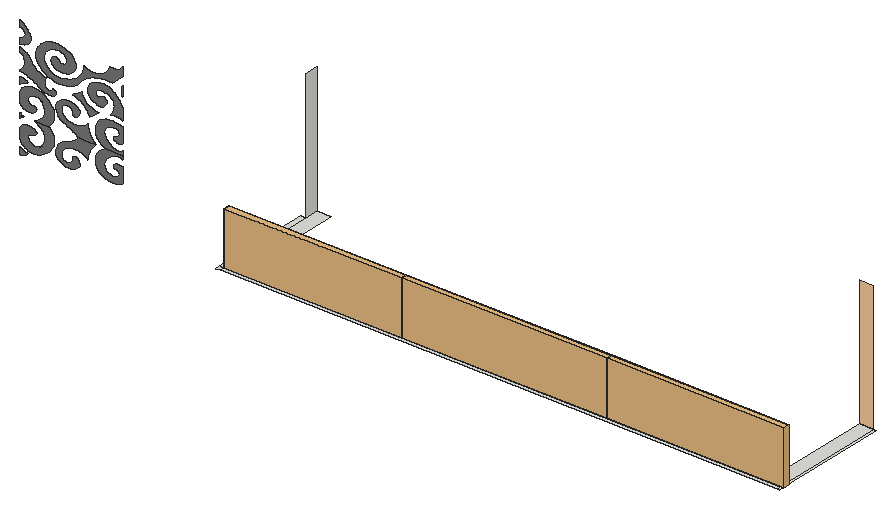
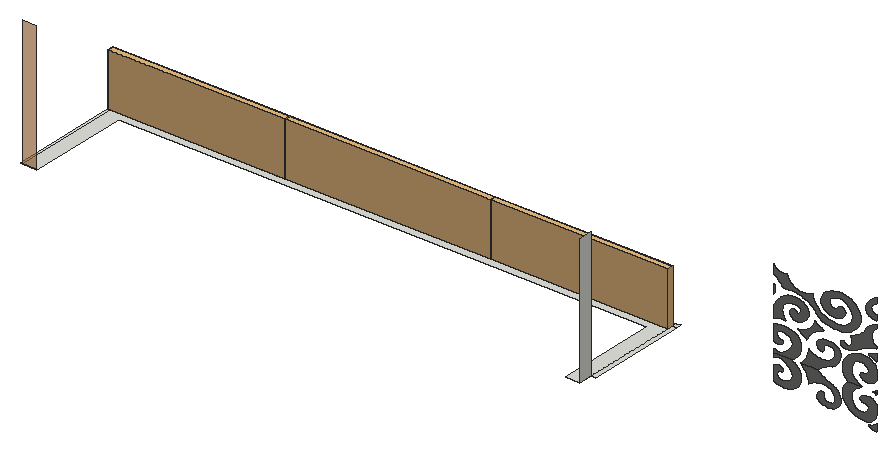
# SketchUp Ruby script. Lengths in inches.
U = 1.inch
M = Sketchup.active_model
def pt(a) = Geom::Point3d.new(a.map { |v| v * U })
def face(e, loops, mat)
  f = e.add_face(loops[0].map { |a| pt(a) })
  loops[1..].each { |l| e.add_face(l.map { |a| pt(a) }).erase! }
  f.material = f.back_material = mat if mat
  f
end
# faces: each face lists its corners as indices into pts; further lists are holes
def faces(e, pts, list, mat = nil) = list.each { |f| face(e, (f[0].is_a?(Array) ? f : [f]).map { |l| l.map { |i| pts[i] } }, mat) }
# xy, xz, yz: faces in a plane at the given z, y or x. An outline is a flat list of corners, or four numbers for a rectangle; further outlines are holes
def ring(l) = l.size == 4 ? [[l[0], l[1]], [l[2], l[1]], [l[2], l[3]], [l[0], l[3]]] : l.each_slice(2).to_a
def flat(e, list, mat, &to3) = list.each { |f| face(e, (f[0].is_a?(Array) ? f : [f]).map { |l| ring(l).map { |u, v| to3.(u, v) } }, mat) }
def xy(e, z, list, mat = nil) = flat(e, list, mat) { |x, y| [x, y, z] }
def xz(e, y, list, mat = nil) = flat(e, list, mat) { |x, z| [x, y, z] }
def yz(e, x, list, mat = nil) = flat(e, list, mat) { |y, z| [x, y, z] }
def lines(e, pts, list) = list.each { |a, b| e.add_line(pt(pts[a]), pt(pts[b])) }
# prism: a flat outline (further loops are holes) pulled along v
def prism(e, loops, v, mat = nil)
  f = face(e, loops, mat); d = Geom::Vector3d.new(v.map { |x| x * U })
  f.pushpull(f.normal.samedirection?(d) ? d.length : -d.length)
end
def box(e, o, s, mat = nil) = prism(e, [[o, [o[0] + s[0], o[1], o[2]], [o[0] + s[0], o[1] + s[1], o[2]], [o[0], o[1] + s[1], o[2]]]], [0, 0, s[2]], mat)
def at(x, y, z, deg = 0) = Geom::Transformation.translation(pt([x, y, z])) * Geom::Transformation.rotation(ORIGIN, Z_AXIS, deg.degrees)
def axes(o, x, y, z) = Geom::Transformation.new([*x, 0, *y, 0, *z, 0, *pt(o).to_a, 1])
def part(name) = M.definitions.add(name)
# library, detail: a bought-in or finely detailed component or shape, given as its bounding box
def library(name, o, s) = part(name).tap { |d| box(d.entities, o, s) }
def detail(e, o, s) = box(e.add_group.entities, o, s)
def put(e, d, t, mat = nil) = e.add_instance(d, t).tap { |i| i.material = mat if mat }
def group(e, t, mat = nil) = e.add_group.tap { |g| g.transformation = t; g.material = mat if mat }.entities
root = M.entities
M.materials.add("[0043_SaddleBrown]4").color = [124, 123, 122]
M.materials.add("[Granite Light Gray]").color = [149, 148, 144]
M.materials.add("[Wood Floor]").color = [224, 152, 88]
M.materials["[Wood Floor]"].alpha = 0.68
c1 = library("Glass Railing",[0,0,0],[139.5,4.76,42])
xy(root,293,[[3049.57,556.4375,3053.01,559.875],[3053.01,556.4375,3491.44,559.875],[3491.44,556.4375,3493.37,559.875],[3049.57,559.875,3053.01,640.11],[3053.01,559.875,3491.44,559.875,3491.44,651.03,3480.11,651.03,3480.11,571.2,3064.33,571.2,3064.33,651.03,3053.01,651.03],
  [3491.44,559.875,3493.37,651.03]])
xz(root,589.17,[[2869.23,295.77,2869.23,301,2869.58,300.64,2869.97,300.3,2870.39,299.98,2870.84,299.68,2871.3125,299.4,2871.8125,299.15,2872.34,298.92,2872.88,298.72,2873.44,298.54,2874.02,298.4,2874.61,298.28,2875.21,298.1875,2874.84,297.86,2874.44,297.54,2874.02,297.25,2873.5625,296.98,2873.08,296.74,2872.58,296.52,2872.05,296.32,2871.51,296.15,2870.96,296.02,2870.39,295.91,2869.81,295.82],[2907.19,299.46,2905.2,299.6,2903.29,300.03,2901.54,300.72,2900.02,301.66,2898.8,302.81,2897.92,304.1,2897.43,305.5,2897.28,306.54,2897.26,307.57,2897.37,308.61,2897.59,309.63,2897.95,310.64,2898.42,311.62,2899.01,312.57,2899.71,313.47,2900.52,314.33,2901.43,315.14,2902.44,315.88,2903.53,316.56,2904.68,316.875,2905.81,317.24,2906.91,317.65,2907.97,318.1,2908.99,318.59,2909.98,319.13,2910.92,319.7,2911.82,320.3125,2912.67,320.96,2913.46,321.64,2914.21,322.35,2914.89,323.09,2928.66,323.09,2927.68,322.2,2926.77,321.27,2925.95,320.31,2925.21,319.31,2924.56,318.28,2924,317.22,2923.53,316.14,2923.15,315.03,2922.86,313.92,2922.68,312.79,2922.58,311.66,2922.59,310.53,2922.01,311.07,2921.375,311.58,2920.69,312.0625,2919.97,312.51,2919.2,312.91,2918.39,313.28,2917.56,313.6,2916.6875,313.88,2915.79,314.11,2914.875,314.3,2913.95,314.44,2913,314.54,2911.375,314.5625,2909.76,314.41,2908.21,314.07,2906.74,313.56,2905.41,312.89,2904.24,312.07,2903.26,311.14,2902.49,310.1,2901.96,308.99,2901.68,307.84,2901.66,306.66,2901.89,305.5,2902.15,304.93,2902.54,304.41,2903.06,303.9375,2903.6875,303.54,2904.4,303.24,2905.1875,303.04,2906.01,302.93,2906.84,302.94,2907.65,303.06,2908.43,303.28,2909.13,303.6,2909.75,304,2909.91,304.24,2910.05,304.5,2910.17,304.75,2910.28,305.01,2910.36,305.28,2910.42,305.54,2910.46,305.8125,2910.49,306.08,2910.49,306.36,2910.47,306.625,2910.43,306.9,2910.37,307.16,2910.33,307.41,2910.36,307.66,2910.44,307.9,2910.58,308.13,2910.77,308.34,2911.01,308.52,2911.29,308.67,2911.6,308.78,2911.93,308.85,2912.28,308.875,2912.62,308.86,2912.96,308.8,2913.56,308.46,2914.12,308.07,2914.6,307.64,2915.02,307.17,2915.37,306.68,2915.64,306.15,2915.83,305.61,2915.94,305.0625,2915.96,304.51,2915.91,303.95,2915.76,303.41,2915.54,302.875,2914.33,301.72,2912.83,300.77,2911.09,300.06,2909.18,299.61],[2880.06,299.94,2878.49,299.97,2876.94,300.16,2875.45,300.52,2874.06,301.04,2872.79,301.7,2871.68,302.5,2870.74,303.41,2870.01,304.41,2869.5,305.48,2869.23,306.59,2869.23,314.54,2869.6875,315.41,2870.37,316.19,2871.24,316.875,2872.27,317.42,2873.43,317.82,2874.68,318.05,2875.96,318.11,2877.23,318,2878.46,317.71,2879.58,317.27,2880.57,316.67,2881.38,315.96,2881.625,315.64,2881.78,315.29,2881.85,314.93,2881.83,314.57,2881.72,314.22,2881.52,313.88,2881.24,313.58,2880.89,313.32,2880.48,313.11,2880.02,312.96,2879.53,312.86,2879.03,312.84,2878.36,312.8,2877.72,312.6875,2877.11,312.49,2876.55,312.23,2876.07,311.89,2875.67,311.51,2875.375,311.08,2875.18,310.62,2875.11,310.14,2875.15,309.66,2875.3,309.1875,2875.56,308.75,2875.94,307.98,2876.51,307.28,2877.26,306.67,2878.15,306.17,2879.16,305.8,2880.24,305.58,2881.37,305.5,2882.49,305.58,2883.57,305.81,2884.57,306.18,2886,307.48,2887.13,308.92,2887.94,310.46,2888.41,312.08,2888.54,313.73,2888.3125,315.38,2887.74,316.98,2886.83,318.5,2885.62,319.9,2884.11,321.15,2882.37,322.22,2880.41,323.09,2891.36,323.09,2893.18,321.23,2894.58,319.18,2895.51,317,2895.95,314.75,2895.89,312.47,2895.34,310.22,2894.3,308.07,2892.8,306.0625,2890.875,304.25,2888.58,302.68,2885.97,301.39,2883.12,300.42,2881.61,300.1],[2941.89,301.35,2939.19,301.57,2936.6,302.17,2934.22,303.12,2932.15,304.39,2930.47,305.93,2929.24,307.67,2928.51,309.5625,2928.31,311.52,2928.65,313.46,2928.73,314.46,2928.93,315.44,2929.26,316.41,2929.71,317.35,2930.28,318.26,2930.96,319.125,2931.74,319.94,2932.63,320.71,2933.61,321.41,2934.68,322.04,2935.82,322.6,2937.02,323.09,2949.62,323.09,2949.62,320.125,2949.32,320.4,2948.97,320.65,2948.59,320.87,2948.17,321.05,2947.73,321.2,2947.27,321.3,2946.79,321.37,2946.31,321.4,2945.82,321.38,2945.34,321.32,2944.87,321.23,2944.42,321.09,2943.34,320.67,2942.31,320.19,2941.32,319.66,2940.4,319.08,2939.53,318.45,2938.72,317.78,2937.99,317.07,2937.33,316.33,2936.75,315.55,2936.24,314.74,2935.82,313.91,2935.48,313.06,2935.28,312.23,2935.25,311.39,2935.39,310.55,2935.7,309.74,2936.16,308.97,2936.78,308.25,2937.53,307.61,2938.4,307.05,2939.38,306.59,2940.4375,306.24,2941.56,306,2942.71,305.875,2943.78,305.92,2944.8,306.14,2945.71,306.54,2946.46,307.09,2947,307.75,2947.29,308.49,2947.33,309.26,2947.11,310.01,2946.64,310.7,2945.95,311.28,2945.09,311.73,2944.1,312.01,2943.85,312,2943.6,312.01,2943.37,312.06,2943.14,312.13,2942.9375,312.23,2942.76,312.36,2942.62,312.5,2942.51,312.66,2942.44,312.83,2942.42,313.01,2942.43,313.18,2942.49,313.36,2942.78,313.84,2943.17,314.28,2943.65,314.67,2944.22,315,2944.85,315.25,2945.53,315.43,2946.24,315.53,2946.97,315.54,2947.6875,315.47,2948.38,315.3125,2949.03,315.08,2949.62,314.77,2949.62,302.99,2947.21,302.08,2944.6,301.53],[2869.23,321.36,2869.23,323.09,2871.62,323.09,2871.31,323.07,2871,323.03,2870.71,322.96,2870.42,322.86,2870.16,322.73,2869.93,322.58,2869.72,322.41,2869.55,322.22,2869.41,322.02,2869.31,321.81,2869.25,321.59],
  [2869.23,323.09,2871.62,323.09,2871.31,323.1,2871,323.15,2870.71,323.22,2870.42,323.32,2870.16,323.45,2869.93,323.59,2869.72,323.76,2869.55,323.95,2869.41,324.16,2869.31,324.37,2869.25,324.59,2869.23,324.82],[2880.41,323.09,2891.36,323.09,2893.18,324.95,2894.58,326.99,2895.51,329.17,2895.95,331.43,2895.89,333.71,2895.34,335.95,2894.3,338.11,2892.8,340.11,2890.875,341.93,2888.58,343.5,2885.97,344.78,2883.12,345.76,2881.61,346.08,2880.06,346.23,2878.49,346.21,2876.94,346.02,2875.45,345.66,2874.06,345.14,2872.79,344.47,2871.68,343.68,2870.74,342.77,2870.01,341.77,2869.5,340.7,2869.23,339.58,2869.23,331.63,2869.6875,330.77,2870.37,329.98,2871.24,329.3,2872.27,328.75,2873.43,328.36,2874.68,328.12,2875.96,328.0625,2877.23,328.18,2878.46,328.46,2879.58,328.91,2880.57,329.5,2881.38,330.22,2881.625,330.54,2881.78,330.88,2881.85,331.24,2881.83,331.61,2881.72,331.96,2881.52,332.29,2881.24,332.6,2880.89,332.86,2880.48,333.07,2880.02,333.22,2879.53,333.3125,2879.03,333.34,2878.36,333.375,2877.72,333.49,2877.11,333.68,2876.55,333.95,2876.07,334.28,2875.67,334.67,2875.375,335.1,2875.18,335.5625,2875.11,336.04,2875.15,336.52,2875.3,336.99,2875.56,337.43,2875.94,338.2,2876.51,338.9,2877.26,339.51,2878.15,340,2879.16,340.375,2880.24,340.6,2881.37,340.68,2882.49,340.6,2883.57,340.37,2884.57,340,2886,338.7,2887.13,337.26,2887.94,335.71,2888.41,334.1,2888.54,332.44,2888.3125,330.8,2887.74,329.2,2886.83,327.68,2885.62,326.28,2884.11,325.02,2882.37,323.95],[2914.89,323.09,2928.66,323.09,2927.68,323.97,2926.77,324.9,2925.95,325.87,2925.21,326.87,2924.56,327.9,2924,328.96,2923.53,330.04,2923.15,331.14,2922.86,332.26,2922.68,333.38,2922.58,334.51,2922.59,335.65,2922.01,335.11,2921.375,334.59,2920.69,334.11,2919.97,333.67,2919.2,333.27,2918.39,332.9,2917.56,332.58,2916.6875,332.3,2915.79,332.0625,2914.875,331.875,2913.95,331.73,2913,331.64,2911.375,331.61,2909.76,331.77,2908.21,332.11,2906.74,332.62,2905.41,333.29,2904.24,334.1,2903.26,335.04,2902.49,336.08,2901.96,337.18,2901.68,338.34,2901.66,339.51,2901.89,340.67,2902.15,341.24,2902.54,341.77,2903.06,342.24,2903.6875,342.63,2904.4,342.9375,2905.1875,343.14,2906.01,343.24,2906.84,343.23,2907.65,343.12,2908.43,342.9,2909.13,342.58,2909.75,342.18,2909.91,341.93,2910.05,341.68,2910.17,341.42,2910.28,341.16,2910.36,340.9,2910.42,340.63,2910.46,340.36,2910.49,340.09,2910.49,339.82,2910.47,339.55,2910.43,339.28,2910.37,339.01,2910.33,338.76,2910.36,338.52,2910.44,338.27,2910.58,338.05,2910.77,337.84,2911.01,337.66,2911.29,337.51,2911.6,337.4,2911.93,337.33,2912.28,337.3,2912.62,337.32,2912.96,337.37,2913.56,337.72,2914.12,338.11,2914.6,338.54,2915.02,339,2915.37,339.5,2915.64,340.02,2915.83,340.5625,2915.94,341.11,2915.96,341.67,2915.91,342.22,2915.76,342.77,2915.54,343.3,2914.33,344.45,2912.83,345.41,2911.09,346.12,2909.18,346.5625,2907.19,346.72,2905.2,346.58,2903.29,346.15,2901.54,345.45,2900.02,344.51,2898.8,343.37,2897.92,342.07,2897.43,340.67,2897.28,339.64,2897.26,338.6,2897.37,337.57,2897.59,336.54,2897.95,335.54,2898.42,334.56,2899.01,333.61,2899.71,332.7,2900.52,331.84,2901.43,331.04,2902.44,330.3,2903.53,329.62,2904.68,329.3,2905.81,328.9375,2906.91,328.53,2907.97,328.08,2908.99,327.58,2909.98,327.05,2910.92,326.47,2911.82,325.86,2912.67,325.22,2913.46,324.54,2914.21,323.83],[2937.02,323.09,2949.62,323.09,2949.62,326.05,2949.32,325.77,2948.97,325.53,2948.59,325.31,2948.17,325.125,2947.73,324.98,2947.27,324.87,2946.79,324.8,2946.31,324.78,2945.82,324.79,2945.34,324.85,2944.87,324.95,2944.42,325.09,2943.34,325.51,2942.31,325.99,2941.32,326.52,2940.4,327.1,2939.53,327.72,2938.72,328.39,2937.99,329.1,2937.33,329.85,2936.75,330.625,2936.24,331.43,2935.82,332.27,2935.48,333.12,2935.28,333.95,2935.25,334.79,2935.39,335.62,2935.7,336.44,2936.16,337.21,2936.78,337.92,2937.53,338.57,2938.4,339.125,2939.38,339.58,2940.4375,339.9375,2941.56,340.18,2942.71,340.3,2943.78,340.26,2944.8,340.03,2945.71,339.64,2946.46,339.09,2947,338.43,2947.29,337.6875,2947.33,336.92,2947.11,336.17,2946.64,335.48,2945.95,334.89,2945.09,334.45,2944.1,334.17,2943.85,334.18,2943.6,334.17,2943.37,334.12,2943.14,334.05,2942.9375,333.95,2942.76,333.82,2942.62,333.68,2942.51,333.52,2942.44,333.35,2942.42,333.17,2942.43,332.99,2942.49,332.82,2942.78,332.34,2943.17,331.9,2943.65,331.51,2944.22,331.18,2944.85,330.92,2945.53,330.74,2946.24,330.65,2946.97,330.64,2947.6875,330.71,2948.38,330.86,2949.03,331.1,2949.62,331.41,2949.62,343.1875,2947.21,344.1,2944.6,344.65,2941.89,344.82,2939.19,344.61,2936.6,344.01,2934.22,343.06,2932.15,341.79,2930.47,340.25,2929.24,338.5,2928.51,336.61,2928.31,334.66,2928.65,332.71,2928.73,331.72,2928.93,330.74,2929.26,329.77,2929.71,328.83,2930.28,327.92,2930.96,327.05,2931.74,326.23,2932.63,325.47,2933.61,324.77,2934.68,324.13,2935.82,323.57],[2923.78,341.21,2924.31,341.68,2924.86,342.15,2925.41,342.61,2925.97,343.0625,2926.54,343.51,2927.12,343.95,2927.71,344.38,2928.3125,344.81,2928.92,345.23,2929.54,345.64,2930.17,346.04,2930.8125,346.4375,2929.14,346.72,2927.53,347.12,2925.98,347.65,2924.52,348.29,2923.17,349.05,2921.9375,349.9,2920.84,350.85,2919.89,351.87,2919.09,352.97,2918.47,354.11,2918.01,355.3,2917.74,356.52,2917.19,356.14,2916.64,355.77,2916.07,355.4,2915.49,355.04,2914.91,354.69,2914.3125,354.35,2913.71,354.02,2913.1,353.6875,2912.48,353.37,2911.22,352.75,2910.58,352.46,2912.18,351.92,2913.72,351.3,2915.1875,350.58,2916.57,349.79,2917.87,348.92,2919.0625,347.98,2920.15,346.98,2921.125,345.91,2921.98,344.8,2922.71,343.64,2923.31,342.4375],
  [2869.23,345.18,2869.58,345.53,2869.97,345.875,2870.39,346.2,2870.84,346.5,2871.3125,346.77,2871.8125,347.03,2872.34,347.26,2872.88,347.46,2873.44,347.63,2874.02,347.78,2874.61,347.9,2875.21,347.99,2874.84,348.32,2874.44,348.63,2874.02,348.93,2873.5625,349.19,2873.08,349.44,2872.58,349.66,2872.05,349.85,2871.51,350.02,2870.96,350.16,2870.39,350.27,2869.81,350.35,2869.23,350.4],[2892.87,345.8,2893.89,345.82,2894.7,345.91,2895.47,346.14,2896.14,346.49,2896.6875,346.93,2897.08,347.45,2897.31,348.03,2897.34,348.625,2897.2,349.21,2896.87,349.76,2896.38,350.24,2895.75,350.625,2895.02,350.9,2894.91,350.3,2894.59,349.75,2894.08,349.27,2893.42,348.9,2892.65,348.67,2891.82,348.59,2890.99,348.67,2890.22,348.9,2889.55,349.27,2889.04,349.75,2888.72,350.3,2888.61,350.9,2888.57,351.375,2888.54,351.85,2888.54,352.33,2888.55,352.8,2888.57,353.28,2888.62,353.75,2888.68,354.22,2888.76,354.7,2888.86,355.17,2888.97,355.63,2889.1,356.1,2889.25,356.5625,2887.79,356.99,2886.38,357.49,2885.03,358.08,2883.74,358.74,2882.54,359.47,2881.42,360.27,2880.39,361.14,2879.45,362.05,2878.625,363.02,2877.91,364.03,2877.3,365.09,2876.82,366.17,2876.29,366.67,2875.75,367.16,2875.18,367.64,2874.59,368.1,2873.98,368.55,2873.36,368.99,2872.71,369.41,2872.05,369.82,2871.37,370.21,2870.67,370.59,2869.95,370.95,2869.23,371.29,2869.23,368.08,2870.24,367.17,2871.1,366.18,2871.78,365.12,2872.27,364.01,2872.57,362.86,2872.67,361.69,2872.57,360.52,2872.27,359.375,2871.78,358.26,2871.1,357.2,2870.24,356.21,2869.23,355.3,2869.23,354.25,2870.51,354.05,2871.78,353.81,2873.04,353.53,2874.27,353.19,2875.47,352.8125,2876.64,352.39,2877.79,351.92,2878.89,351.4,2879.96,350.85,2880.99,350.26,2881.97,349.63,2882.9,348.96,2883.63,348.45,2884.41,347.98,2885.23,347.55,2886.09,347.16,2886.99,346.82,2887.92,346.53,2888.875,346.28,2889.85,346.08,2890.85,345.9375,2891.86,345.85],[2949.62,347.78,2949.62,356.71,2949.25,357.36,2948.87,358,2948.48,358.64,2948.0625,359.27,2947.64,359.9,2947.2,360.52,2946.74,361.13,2946.27,361.74,2945.78,362.35,2945.28,362.95,2944.76,363.54,2944.23,364.12,2943.375,364.94,2942.39,365.6875,2941.3,366.34,2940.1,366.9,2938.83,367.36,2937.49,367.71,2936.1,367.94,2934.6875,368.0625,2933.26,368.0625,2931.85,367.94,2930.46,367.71,2929.12,367.36,2927.1875,366.59,2925.49,365.57,2924.11,364.33,2923.07,362.92,2922.44,361.39,2922.23,359.81,2922.44,358.23,2923.07,356.7,2924.11,355.29,2925.49,354.05,2927.1875,353.03,2929.12,352.26,2929.76,351.99,2930.46,351.8,2931.18,351.6875,2931.92,351.66,2932.66,351.71,2933.38,351.86,2934.06,352.08,2934.68,352.37,2935.23,352.73,2935.6875,353.15,2936.05,353.62,2936.31,354.12,2936.67,354.57,2936.95,355.05,2937.125,355.55,2937.2,356.0625,2937.18,356.58,2937.05,357.09,2936.83,357.59,2936.51,358.05,2936.1,358.48,2935.62,358.86,2935.0625,359.19,2934.45,359.46,2934.09,359.32,2933.75,359.17,2933.43,359,2933.12,358.82,2932.83,358.62,2932.56,358.41,2932.31,358.18,2932.08,357.94,2931.875,357.69,2931.69,357.43,2931.54,357.17,2931.41,356.89,2930.65,357.23,2929.98,357.65,2929.44,358.17,2929.03,358.74,2928.79,359.36,2928.7,360,2928.79,360.64,2929.03,361.26,2929.44,361.84,2929.98,362.35,2930.65,362.78,2931.41,363.11,2932.34,363.13,2933.28,363.11,2934.2,363.03,2935.12,362.91,2936.02,362.73,2936.91,362.51,2937.76,362.24,2938.59,361.93,2939.38,361.57,2940.13,361.17,2940.84,360.73,2941.5,360.26,2942.09,359.34,2942.55,358.39,2942.9,357.41,2943.125,356.41,2943.22,355.41,2943.19,354.4,2943.04,353.39,2942.76,352.4,2942.36,351.4375,2941.84,350.5,2941.21,349.6,2940.46,348.74,2941.23,348.93,2942.01,349.07,2942.8,349.17,2943.61,349.21,2944.41,349.2,2945.22,349.14,2946.01,349.03,2946.79,348.875,2947.54,348.67,2948.27,348.42,2948.96,348.12],[2899.9,356.35,2903.06,356.47,2906.14,356.98,2909.0625,357.86,2911.74,359.07,2914.09,360.6,2916.04,362.39,2916.58,363.14,2917.17,363.86,2917.81,364.5625,2918.49,365.25,2919.22,365.9,2919.98,366.53,2920.79,367.14,2921.64,367.72,2922.52,368.26,2923.44,368.78,2924.39,369.26,2925.375,369.72,2926.68,370.16,2928.01,370.56,2929.375,370.9,2930.76,371.18,2932.17,371.41,2933.59,371.59,2935.02,371.7,2936.46,371.76,2937.9,371.77,2939.34,371.71,2940.78,371.6,2942.2,371.43,2943.32,372.71,2943.9,373.34,2944.49,373.96,2945.1,374.58,2945.71,375.19,2946.33,375.8,2946.97,376.4,2947.61,376.99,2948.27,377.58,2948.9375,378.16,2949.62,378.74,2949.62,385.48,2949.25,384.78,2948.75,384.13,2948.13,383.54,2947.4,383.01,2946.58,382.5625,2945.68,382.2,2944.71,381.9375,2943.7,381.77,2942.68,381.71,2941.65,381.75,2940.63,381.9,2939.66,382.14,2939.22,380.54,2938.4,379.02,2937.24,377.62,2935.76,376.38,2934.01,375.35,2932.04,374.54,2929.91,373.99,2927.68,373.7,2925.41,373.7,2923.18,373.98,2921.04,374.52,2919.07,375.32,2919.01,373.3,2918.54,371.31,2917.68,369.39,2916.4375,367.57,2914.85,365.91,2912.93,364.43,2910.75,363.17,2908.33,362.14,2905.73,361.39,2903,360.91,2900.21,360.72,2897.41,360.82,2894.96,361.55,2892.75,362.6,2890.86,363.94,2889.36,365.52,2888.32,367.27,2887.76,369.14,2887.72,371.05,2888.1875,372.94,2889.15,374.72,2890.57,376.33,2892.4,377.71,2894.5625,378.82,2895.96,379.26,2897.45,379.49,2898.97,379.5,2900.47,379.28,2901.87,378.85,2903.12,378.22,2904.17,377.42,2904.96,376.48,2905.48,375.45,2905.69,374.36,2905.6,373.26,2905.19,372.2,2904.91,371.81,2904.54,371.47,2904.07,371.19,2903.54,370.98,2902.96,370.85,2902.36,370.81,2901.75,370.85,2901.17,370.98,2900.64,371.19,2900.18,371.47,2899.8,371.81,2899.52,372.2,2899.39,372.43,2899.23,372.65,2899.04,372.85,2898.83,373.05,2898.6,373.23,2898.35,373.4,2898.08,373.55,2897.8,373.6875,2897.5,373.81,2897.18,373.91,2896.86,373.99,2896.53,374.05,2895.95,373.81,2895.42,373.51,2894.94,373.17,2894.52,372.79,2894.16,372.37,2893.89,371.93,2893.68,371.47,2893.5625,370.99,2893.52,370.5,2893.57,370.02,2893.69,369.54,2893.9,369.08,2894.29,368.45,2894.77,367.87,2895.33,367.32,2895.98,366.82,2896.69,366.37,2897.47,365.98,2898.3,365.65,2899.17,365.39,2900.08,365.2,2901.01,365.08,2901.95,365.03,2902.9,365.05,2904.39,365.22,2905.84,365.53,2907.22,365.98,2908.5,366.56,2909.66,367.25,2910.69,368.05,2911.55,368.95,2912.25,369.91,2912.76,370.9375,2913.07,372,2913.1875,373.09,2913.1,374.18,2912.5,375.81,2911.57,377.37,2910.35,378.8125,2908.86,380.12,2907.13,381.26,2905.1875,382.21,2903.08,382.95,2900.85,383.47,2898.53,383.76,2896.1875,383.8,2893.85,383.61,2891.59,383.18,2889.39,382.09,2887.41,380.8125,2885.67,379.36,2884.22,377.75,2883.06,376.03,2882.22,374.21,2881.71,372.32,2881.55,370.41,2881.73,368.5,2882.25,366.62,2883.11,364.8,2884.29,363.08,2886.09,361.21,2888.31,359.58,2890.88,358.25,2893.72,357.25,2896.76,356.61],[2949.62,364.66,2949.62,371.94,2949.39,371.35,2949.21,370.75,2949.0625,370.14,2948.96,369.53,2948.9,368.92,2948.875,368.3,2948.9,367.69,2948.96,367.07,2949.0625,366.46,2949.21,365.85,2949.39,365.25],
  [2869.23,373.83,2870.47,373.9,2871.69,374.11,2872.86,374.45,2873.93,374.91,2874.9,375.49,2875.74,376.16,2876.42,376.92,2876.9375,377.74,2877.28,378.61,2877.43,379.51,2877.39,380.41,2877.16,381.3,2876.8125,382.16,2876.4,383.01,2875.93,383.84,2875.4,384.65,2874.81,385.45,2874.16,386.22,2873.47,386.96,2872.71,387.68,2871.91,388.36,2871.0625,389.02,2870.17,389.64,2869.23,390.23,2869.23,385.49,2870.31,385.16,2871.27,384.67,2872.07,384.05,2872.67,383.32,2873.04,382.52,2873.17,381.67,2873.04,380.83,2872.67,380.02,2872.07,379.29,2871.27,378.67,2870.31,378.18,2869.23,377.85]],"[0043_SaddleBrown]4")
xz(root,651.03,[[3480.11,293,3491.44,394.4375]],"[Wood Floor]")
yz(root,3053.01,[[640.11,293,651.03,394.4375]])
p = [[2884.57,589.17,306.18],[2885.46,589.17,306.68],[2886.21,589.17,307.29],[2884.57,589.17,340],[2885.46,589.17,339.5],[2886.21,589.17,338.89]]
lines(root,p,[[0,1],[1,2],[3,4],[4,5]])
put(root,c1,at(3053.01,559.875,293))
put(root,c1,axes([3192.51,559.875,293],[1.15726,0,0],[0,1,0],[0,0,1]),"[Granite Light Gray]")
put(root,c1,at(3353.95,559.875,293))
